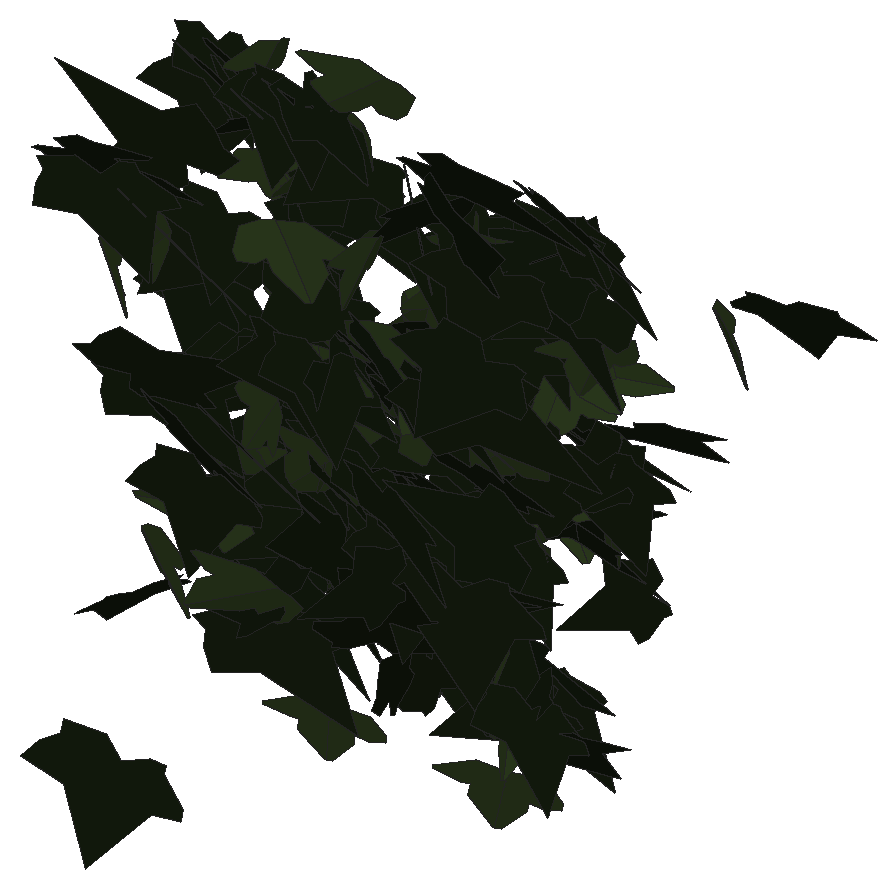
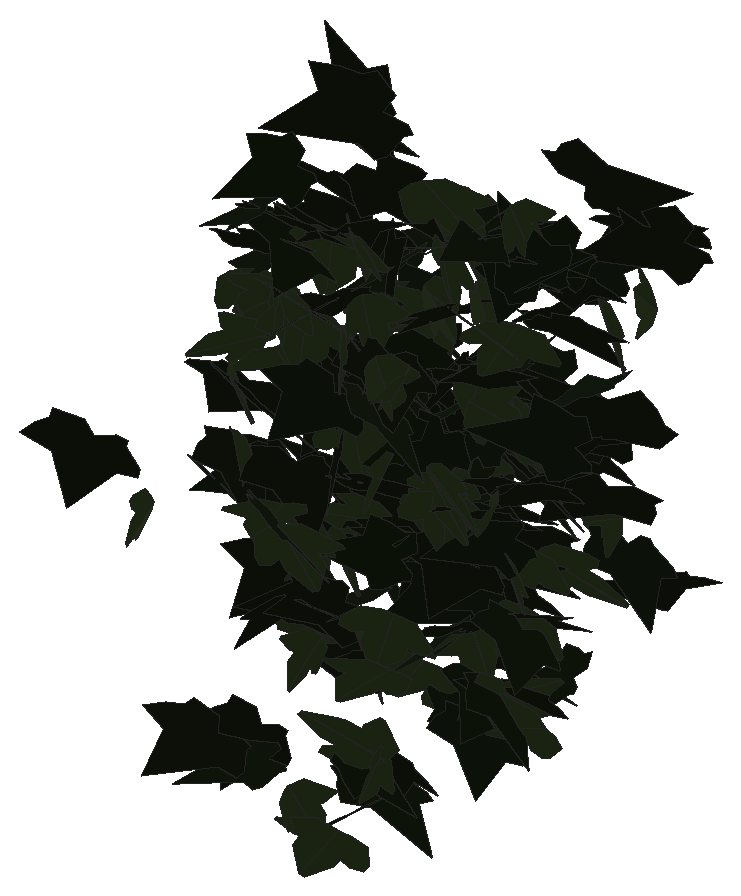
# SketchUp Ruby script. Lengths in millimetres.
U = 1.mm
M = Sketchup.active_model
def pt(a) = Geom::Point3d.new(a.map { |v| v * U })
def face(e, loops, mat)
  f = e.add_face(loops[0].map { |a| pt(a) })
  loops[1..].each { |l| e.add_face(l.map { |a| pt(a) }).erase! }
  f.material = f.back_material = mat if mat
  f
end
# faces: each face lists its corners as indices into pts; further lists are holes
def faces(e, pts, list, mat = nil) = list.each { |f| face(e, (f[0].is_a?(Array) ? f : [f]).map { |l| l.map { |i| pts[i] } }, mat) }
# xy, xz, yz: faces in a plane at the given z, y or x. An outline is a flat list of corners, or four numbers for a rectangle; further outlines are holes
def ring(l) = l.size == 4 ? [[l[0], l[1]], [l[2], l[1]], [l[2], l[3]], [l[0], l[3]]] : l.each_slice(2).to_a
def flat(e, list, mat, &to3) = list.each { |f| face(e, (f[0].is_a?(Array) ? f : [f]).map { |l| ring(l).map { |u, v| to3.(u, v) } }, mat) }
def xy(e, z, list, mat = nil) = flat(e, list, mat) { |x, y| [x, y, z] }
def xz(e, y, list, mat = nil) = flat(e, list, mat) { |x, z| [x, y, z] }
def yz(e, x, list, mat = nil) = flat(e, list, mat) { |y, z| [x, y, z] }
def lines(e, pts, list) = list.each { |a, b| e.add_line(pt(pts[a]), pt(pts[b])) }
# prism: a flat outline (further loops are holes) pulled along v
def prism(e, loops, v, mat = nil)
  f = face(e, loops, mat); d = Geom::Vector3d.new(v.map { |x| x * U })
  f.pushpull(f.normal.samedirection?(d) ? d.length : -d.length)
end
def box(e, o, s, mat = nil) = prism(e, [[o, [o[0] + s[0], o[1], o[2]], [o[0] + s[0], o[1] + s[1], o[2]], [o[0], o[1] + s[1], o[2]]]], [0, 0, s[2]], mat)
def at(x, y, z, deg = 0) = Geom::Transformation.translation(pt([x, y, z])) * Geom::Transformation.rotation(ORIGIN, Z_AXIS, deg.degrees)
def axes(o, x, y, z) = Geom::Transformation.new([*x, 0, *y, 0, *z, 0, *pt(o).to_a, 1])
def part(name) = M.definitions.add(name)
# library, detail: a bought-in or finely detailed component or shape, given as its bounding box
def library(name, o, s) = part(name).tap { |d| box(d.entities, o, s) }
def detail(e, o, s) = box(e.add_group.entities, o, s)
def put(e, d, t, mat = nil) = e.add_instance(d, t).tap { |i| i.material = mat if mat }
def group(e, t, mat = nil) = e.add_group.tap { |g| g.transformation = t; g.material = mat if mat }.entities
root = M.entities
M.materials.add("efeu1").color = [18, 25, 13]
M.materials.add("efeu2").color = [43, 57, 29]
c1 = part("ivyleaf_10")
p = [[0,12.8,-0.8],[-1.5,51.3,-10.9],[-4.9,51,-11.6],[-13.6,26.5,-7.3],[-13.2,15.9,-4.6],[-21.1,19.3,-7.2],
  [-29.5,16.3,-8.3],[-29.2,8.3,-6.2],[-19.7,-9.8,0.5],[-7.6,-13,4],[1,-12.2,5.8],[-0.4,51.1,-11.1],
  [-1.5,51.1,-10.9],[1,-12.4,5.9],[16.9,-12.4,3.5],[35.1,9.1,-5.1],[35,12.9,-6.1],[20.5,16.4,-4.9],
  [15.8,15,-3.8],[15.3,27.6,-7.1],[12.8,31.3,-7.8]]
faces(c1.entities,p,[[0,1,2,3,4,5,6,7,8,9,10],[11,12,0,13,14,15,16,17,18,19,20]],"efeu2")
c2 = part("ivyleaf_9")
p = [[39.1,54.8,31.7],[34.5,51.8,30.2],[-5.3,25.2,17.3],[-17.9,28.3,20.9],[-21.6,21.7,17],[-20.2,4.3,5.3],
  [-22.9,-0.3,2.5],[-17.1,-4,-0.6],[-2,-2.1,-1.2],[-0.7,-15.4,-10.1],[16.6,-22.3,-16.7],[21.1,-15.1,-12.5],
  [32.7,-10.7,-11],[46.1,-1.8,-6.6],[30.8,11.2,3.8]]
faces(c2.entities,p,[[0,1,2,3,4,5,6,7,8,9,10,11,12,13,14]],"efeu1")
put(root,c1,axes([6232.5,1056.6,3614.3],[-0.05301,-0.61059,-0.9805],[0.31818,0.96833,-0.60776],[2.1752,-0.15652,0.06501]))
put(root,c2,axes([6249.3,764.1,3661.4],[0.62349,1.03972,0.40292],[-0.08884,0.43237,-1.07776],[-2.12033,0.28762,0.16364]))
put(root,c2,axes([6209.3,719.3,3591.9],[1.27144,-0.98934,0.14029],[0.12142,-0.12619,-1.19365],[1.89788,0.67086,-0.01762]))
put(root,c2,axes([6208.7,511.3,4104.5],[2.12507,0.22385,0.53376],[0.99329,0.11205,-1.13878],[-0.47626,1.23251,0.00658]))
put(root,c2,axes([6232.9,713.1,4143.1],[0.08178,-1.24795,-0.07814],[-0.03089,0.07763,-1.24862],[2.37956,0.04389,-0.01352]))
put(root,c2,axes([6218.2,708.4,3903.7],[1.22381,0.07724,1.11184],[1.74203,0.69576,-0.57771],[-1.21021,1.07962,0.29276]))
put(root,c2,axes([6249.1,685.7,3888.7],[-1.16287,-1.04199,0.06481],[0.13254,-0.11561,-1.20211],[1.98252,-0.60346,0.11838]))
put(root,c1,axes([6275.1,773.1,3563.5],[0.97003,0.62714,0.84354],[-1.0128,-0.6545,0.80813],[1.72518,-0.73686,0.00013]))
put(root,c2,axes([6228.3,627.8,3807.5],[-0.63659,-0.70921,-1.06674],[1.06415,0.9111,-0.78106],[2.19345,-0.64785,0.06934]))
put(root,c1,axes([6217.4,778.9,3544.9],[1.27917,-0.07652,0.94431],[1.79881,0.13391,-0.66186],[-0.1242,1.15131,0.13975]))
put(root,c2,axes([6258.2,1022.9,3608.5],[-1.9163,-0.03935,-0.6563],[1.24656,0.04446,-1.00753],[0.10893,-1.20107,-0.0158]))
put(root,c1,axes([6272.5,569.3,4006.5],[0.92456,-0.93891,-0.66939],[-0.43427,0.63373,-1.05449],[2.15118,0.53147,0.07482]))
put(root,c2,axes([6261.3,690.1,4122.7],[-1.8784,-0.64082,-0.43417],[0.80372,0.14384,-1.17228],[1.23462,-1.06861,0.10257]))
put(root,c2,axes([6282,772.7,3572.1],[-0.28697,1.1485,-0.09498],[0.04934,-0.09239,-1.15827],[-2.19272,-0.15238,-0.01363]))
put(root,c2,axes([6286.9,742.7,3658.5],[-1.79291,-0.44896,0.52127],[-0.65172,-0.46059,-1.01555],[1.13559,-0.97316,0.24017]))
put(root,c2,axes([6283.4,1045,3602.5],[-0.96373,0.75103,-0.72225],[0.4298,-0.70483,-0.89125],[-1.93594,-0.53035,0.16168]))
put(root,c1,axes([6302.6,629.6,3679],[0.87197,-0.10124,-1.08289],[-1.99972,0.26228,-0.46907],[0.5346,1.1462,0.01169]))
put(root,c1,axes([6260.9,740.5,3660.5],[-2.08189,0.17325,-0.34606],[0.63339,-0.10845,-1.10628],[-0.37593,-1.14219,0.05255]))
put(root,c1,axes([6272.1,757.5,3744.2],[1.12472,-1.03315,-0.04774],[0.08934,0.08172,-1.18745],[1.96635,0.58723,0.08126]))
put(root,c2,axes([6274.2,720.4,3839.9],[-1.10481,-1.02823,0.31517],[-0.2383,-0.2911,-1.18032],[2.03287,-0.59294,0.03293]))
put(root,c1,axes([6253.6,514.3,4002.3],[-0.29737,0.54425,-1.13301],[0.71097,-1.07003,-0.56551],[-2.28413,-0.40392,-0.02852]))
put(root,c2,axes([6250.1,666.7,4146],[2.24581,-0.45086,-0.2997],[-0.51361,0.1332,-1.26292],[0.89322,1.21017,0.02735]))
put(root,c2,axes([6262.3,633.6,3925.4],[-0.58984,-1.05015,0.63585],[0.11524,-0.66807,-1.07386],[2.33362,-0.23244,0.21375]))
put(root,c2,axes([6270.5,771.7,3577.5],[-1.45641,-0.65826,-0.57461],[0.85524,0.35858,-1.00924],[1.42619,-0.88724,0.01843]))
put(root,c1,axes([6253.9,1055.6,3623.5],[-0.9404,-0.48923,0.92476],[1.29808,0.62487,0.69501],[-1.50983,0.84195,0.02154]))
put(root,c1,axes([6260.3,1115.5,3524.7],[2.02857,0.20437,0.47791],[0.70398,0.46776,-1.025],[-0.69497,1.07036,0.35669]))
put(root,c2,axes([6262.4,491.6,4101.6],[-0.88382,-0.92601,-0.72646],[0.85052,0.58375,-1.02977],[2.07225,-0.63454,0.11281]))
put(root,c2,axes([6299.4,495.2,3642.6],[0.21417,1.25654,-0.14344],[-0.03367,-0.14242,-1.26156],[-2.40674,0.11381,0.00488]))
put(root,c2,axes([6246.5,565.1,3841.8],[0.08093,-0.25758,1.32814],[2.51797,-0.26974,-0.09467],[0.53802,1.30115,0.24329]))
put(root,c2,axes([6278.9,727.1,3837.3],[-1.05285,-0.9828,-0.49121],[0.82274,0.31091,-1.1089],[1.92242,-0.67131,0.20556]))
put(root,c2,axes([6341.6,517.9,4138.5],[-0.04794,0.02741,1.38699],[-2.13929,0.8126,-0.03647],[-1.54735,-1.12431,0.00745]))
put(root,c2,axes([6304,773.3,3510.7],[0.68411,1.10542,0.12641],[-0.015,0.13537,-1.16136],[-2.1175,0.35618,0.04906]))
put(root,c2,axes([6318.5,613.4,4000.6],[-2.21471,-0.36537,0.03234],[-0.0571,-0.0124,-1.21968],[0.69574,-1.16406,0.00284]))
put(root,c2,axes([6300.2,745.1,3705.3],[-1.90049,-0.35101,-0.50364],[0.92645,0.13317,-1.05797],[0.71185,-1.11043,0.03232]))
put(root,c2,axes([6285.9,1050.6,3522.3],[-0.00059,-1.1861,0.07634],[-0.02876,-0.07633,-1.18601],[2.26188,-0.00128,-0.01506]))
put(root,c2,axes([6325.9,673.5,3826.8],[-2.07058,0.44277,-0.26856],[0.47756,-0.09588,-1.17458],[-0.86215,-1.11649,-0.00563]))
put(root,c2,axes([6345.5,732.4,3594.6],[-1.88833,0.31067,0.52272],[-0.92657,0.1935,-1.0391],[-0.69339,-1.10464,-0.03501]))
put(root,c2,axes([6269.8,708.5,4118.2],[2.25595,-0.48028,-0.56029],[1.04081,-0.14012,1.27708],[-0.94304,-1.30358,0.06916]))
put(root,c1,axes([6300.3,719.8,4032.5],[-1.77868,-0.71839,-0.39001],[0.91882,-0.00703,-1.1439],[1.25543,-1.01266,0.28462]))
put(root,c2,axes([6310.8,744.9,3549.7],[0.75041,0.9439,0.60512],[0.35622,0.57703,-1.02204],[-2.10394,0.43436,0.04278]))
put(root,c1,axes([6306.3,693,3710.8],[-2.12167,-0.29345,-0.3124],[0.59799,0.03256,-1.15182],[0.55482,-1.15728,0.04681]))
put(root,c1,axes([6312,775.4,3632.8],[1.17688,0.9457,-0.28185],[-0.5072,-0.16021,-1.12226],[-1.8083,0.66042,0.13134]))
put(root,c1,axes([6314.7,689.2,4175.6],[-0.25923,-1.20094,0.332],[0.19943,-0.34384,-1.20076],[2.36296,-0.10273,0.13776]))
put(root,c2,axes([6276.5,752,3774.6],[2.17748,-0.26341,0.18836],[0.33859,-0.06662,-1.17379],[0.51497,1.1576,-0.02469]))
put(root,c2,axes([6342.1,928.3,3495.4],[-0.01489,1.13626,-0.24426],[-0.89474,-0.22648,-1.03851],[-2.02289,0.09181,0.46114]))
put(root,c1,axes([6307.4,751.8,3806.7],[-0.32943,1.14607,-0.2796],[0.04214,-0.27939,-1.15891],[-2.24478,-0.17343,0.01927]))
put(root,c1,axes([6325.1,1101.8,3551.6],[-0.34351,-1.11285,0.38624],[-0.00678,-0.39023,-1.12601],[2.2419,-0.1717,0.05578]))
put(root,c2,axes([6281.2,536.1,4046.4],[1.4568,-0.93345,0.51682],[0.63787,-0.39351,-1.20713],[1.92789,0.83556,0.00886]))
put(root,c2,axes([6319,617.5,4021.5],[-0.72037,-1.14315,0.21033],[-0.13577,-0.19794,-1.20417],[2.20799,-0.38513,-0.00542]))
put(root,c2,axes([6330.6,667,4115.8],[1.101,1.10722,0.09654],[0.07566,0.08815,-1.24923],[-2.11391,0.57984,0.00557]))
put(root,c1,axes([6309.9,517.9,3690.6],[-0.95877,0.74151,-0.88779],[0.83749,-0.77267,-0.89506],[-2.03595,-0.66703,0.0499]))
put(root,c2,axes([6338.6,752.5,3787.1],[-1.60733,-0.82833,-0.18309],[0.36491,0.06528,-1.17978],[1.57275,-0.86169,0.08662]))
put(root,c2,axes([6362.7,672.8,3674.6],[-1.9795,-0.59,0.39192],[-0.65357,-0.18893,-1.19577],[1.17902,-1.09531,-0.00485]))
put(root,c2,axes([6345,774.3,3638.7],[-0.9698,-1.0459,0.04124],[0.04507,-0.05737,-1.1625],[1.99159,-0.508,0.04639]))
put(root,c2,axes([6309.1,545.4,3811.1],[1.01793,-0.74557,0.84956],[0.85177,-0.72337,-0.91658],[1.9754,0.6961,-0.04256]))
put(root,c1,axes([6359.5,700.7,4056.8],[-0.0824,-1.22848,-0.26768],[-0.06577,0.2689,-1.22849],[2.39199,-0.03493,-0.043]))
put(root,c2,axes([6344.7,675.1,4139.3],[-0.71835,-1.16583,0.13824],[-0.10992,-0.1266,-1.2253],[2.23165,-0.38151,-0.01585]))
put(root,c1,axes([6359.6,700.8,3901.9],[-0.42811,-0.75898,0.99529],[0.03203,-1.01298,-0.76866],[2.38195,-0.12279,0.18922]))
put(root,c1,axes([6380,757.4,3822.3],[0.79364,-0.5299,-0.96676],[-1.16785,0.74714,-0.67421],[1.74315,0.74182,-0.01154]))
put(root,c2,axes([6326.9,730.9,3684.3],[1.85925,-0.6502,-0.05486],[-0.10712,0.01444,-1.17335],[1.23722,0.97834,-0.01915]))
put(root,c1,axes([6349.7,719,3696.6],[-2.10011,-0.11334,-0.39142],[0.77218,-0.20025,-1.08581],[0.07229,-1.15358,0.22694]))
put(root,c2,axes([6354.3,747.7,3723],[1.97838,0.39973,-0.36048],[-0.64775,-0.11925,-1.11366],[-0.79365,1.09375,0.01033]))
put(root,c1,axes([6394.9,754.1,3806.4],[-1.49231,0.27745,0.8565],[-1.5876,0.20341,-0.82956],[-0.64463,-1.14326,0.06026]))
put(root,c2,axes([6395.1,688.1,4006.1],[0.2398,0.73833,0.99377],[-1.25297,0.88592,-0.57473],[-1.99545,-0.46755,0.48031]))
put(root,c2,axes([6343.1,776,3631],[1.3619,-0.63693,-0.66418],[-0.53594,0.64944,-0.92618],[1.66737,0.72899,0.2448]))
put(root,c2,axes([6352.5,668.6,4137.1],[1.40171,0.63723,0.79432],[0.57405,0.79981,-0.92129],[-1.85114,0.73054,0.31578]))
put(root,c2,axes([6343,713.3,3987.7],[0.61839,-1.16376,-0.32096],[-0.07963,0.32133,-1.20745],[2.29618,0.32456,0.04457]))
put(root,c2,axes([6338.8,769.9,3532.9],[0.51879,-0.89059,0.71161],[0.42236,-0.67621,-0.93131],[2.12809,0.35132,0.01136]))
put(root,c1,axes([6379.5,754.8,3785.1],[-1.97198,-0.54972,0.0504],[-0.08195,-0.02636,-1.17293],[1.04741,-1.03703,0.0031]))
put(root,c2,axes([6368.7,383.8,3521.1],[-1.4246,-1.25737,0.03019],[-0.02962,-0.02587,-1.46331],[2.39353,-0.74869,-0.00014]))
put(root,c2,axes([6366.9,524.2,3780.6],[-1.96974,-0.27354,-0.73194],[1.38995,0.09326,-1.06754],[0.52874,-1.26419,0.07962]))
put(root,c2,axes([6361.5,679.2,4142],[-0.33676,-1.16768,0.36339],[0.22932,-0.38204,-1.16892],[2.31614,-0.13195,0.16857]))
put(root,c2,axes([6375.1,689.4,3832.4],[-0.91054,-0.05091,1.13101],[0.10556,-1.22742,-0.03179],[2.15212,0.03867,0.48008]))
put(root,c2,axes([6402.9,683.2,3931.5],[-1.91895,-0.64966,0.29713],[-0.40501,-0.21748,-1.19766],[1.29788,-1.0284,0.06557]))
put(root,c1,axes([6425,729.5,3765.6],[0.67534,0.16747,-1.12453],[-2.06941,0.39415,-0.28441],[0.63215,1.11137,0.27032]))
put(root,c1,axes([6391.5,589.5,3842.8],[1.44432,-0.96288,-0.33665],[-0.22499,0.33376,-1.22107],[1.92825,0.76017,0.10969]))
put(root,c1,axes([6394.6,707.9,3790.8],[0.03269,-1.10472,-0.47812],[0.18426,0.47789,-1.1007],[2.28354,-0.02275,0.09566]))
put(root,c1,axes([6399.1,705.8,3674.1],[0.08549,-1.17309,0.03024],[-0.02074,-0.03068,-1.17388],[2.23326,0.04462,-0.01206]))
put(root,c2,axes([6369.5,681.2,4150.1],[0.89883,-1.11192,-0.44039],[-0.17361,0.43862,-1.20526],[2.26951,0.47392,0.08222]))
put(root,c2,axes([6371.2,684.3,3763.8],[0.31078,-1.15416,0.38697],[0.20438,-0.37526,-1.16454],[2.30774,0.18866,0.05102]))
put(root,c1,axes([6431.3,704.7,4174.5],[-1.73617,-0.42045,0.7532],[-1.19273,-0.43024,-0.9992],[1.1281,-1.10199,0.10274]))
put(root,c1,axes([6421.4,1003,3832.9],[-1.47331,-0.79521,0.40229],[-0.55209,-0.27901,-1.10971],[1.60371,-0.82659,-0.01244]))
put(root,c2,axes([6375.4,718.4,3650.3],[2.04658,0.33696,0.32128],[0.53682,0.17182,-1.12429],[-0.70496,1.10907,0.07657]))
put(root,c2,axes([6381.9,697.6,3674.5],[-0.71118,-0.70522,-0.99888],[0.80653,0.90505,-0.79751],[2.18288,-0.56416,-0.03077]))
put(root,c2,axes([6372.6,1106,3590.8],[2.02981,-0.48671,-0.23478],[-0.01487,0.50552,-1.08345],[1.02834,0.96801,0.44776]))
put(root,c1,axes([6415.4,662.2,3471.5],[-2.08781,-0.40835,0.09557],[-0.1608,-0.04696,-1.17044],[0.7818,-1.10015,0.01448]))
put(root,c1,axes([6404.3,713.4,4103.5],[1.63278,-0.86703,-0.27942],[0.03187,0.39878,-1.18597],[1.73342,0.80936,0.285]))
put(root,c2,axes([6441.8,674.4,3746.6],[-2.05619,-0.45228,0.729],[-1.27776,-0.28408,-1.17123],[1.01648,-1.272,0.00237]))
put(root,c1,axes([6437,625.3,3778.1],[-1.80419,0.22178,0.68669],[-1.31132,0.05878,-0.97016],[-0.4082,-1.16908,0.08149]))
put(root,c2,axes([6412.9,615.5,3879],[0.82511,-1.18761,-0.69133],[0.4202,-0.6553,1.26418],[-2.58136,-0.48628,-0.01519]))
put(root,c2,axes([6384.9,713.9,4042],[0.29901,-1.07885,-0.60291],[0.28765,0.61997,-1.07],[2.33449,0.06179,0.20907]))
put(root,c2,axes([6412.2,713.4,3852.7],[1.7619,-0.09633,-0.76545],[-1.4253,0.17504,-0.92776],[0.35275,1.18841,0.0746]))
put(root,c2,axes([6411.4,1070,3607.6],[2.06853,0.01255,-0.51831],[-0.98673,0.01986,-1.08669],[-0.00529,1.20397,0.02333]))
put(root,c2,axes([6434.4,691.7,4096.6],[-1.73442,-0.67348,0.51749],[-0.27302,-0.62605,-1.0674],[1.59323,-0.84045,0.38043]))
put(root,c2,axes([6386,519.7,3853.7],[1.86849,-0.79741,0.12429],[0.19887,-0.06849,-1.26473],[1.52302,0.98723,0.01266]))
put(root,c1,axes([6425.8,801.5,3625],[-2.19935,-0.0944,-0.0961],[0.18266,0.00549,-1.15945],[0.17991,-1.15958,0.00233]))
put(root,c2,axes([6398.2,637.9,3613.2],[0.93623,-1.17285,-0.11904],[-0.06194,0.11542,-1.27175],[2.24277,0.49279,0.01457]))
put(root,c1,axes([6429.8,645,3787.6],[0.36199,-0.93641,-0.81977],[0.19376,0.83821,-0.93386],[2.36066,0.07479,0.20235]))
put(root,c1,axes([6433.2,686.2,3651.2],[-0.05527,-1.13651,-0.47139],[0.1245,0.46942,-1.13581],[2.33836,-0.05186,0.04933]))
put(root,c1,axes([6407.2,765,3558],[2.00634,0.29448,0.43772],[0.7854,0.14904,-1.09413],[-0.62551,1.13168,0.0302]))
put(root,c2,axes([6382.1,695.5,3680.8],[1.48132,-0.17336,0.99952],[1.84203,-0.25047,-0.79712],[0.57834,1.24181,-0.02124]))
put(root,c2,axes([6461.8,1002.5,3863.5],[-1.68716,0.77661,-0.13606],[0.18098,-0.09793,-1.1785],[-1.4896,-0.8915,0.01093]))
put(root,c2,axes([6482.2,696.3,3656],[-0.67156,0.28688,1.16377],[-1.83672,0.65147,-0.45321],[-1.35289,-1.02687,0.0376]))
put(root,c1,axes([6417.7,636.1,3883],[2.19798,-0.21825,0.33949],[0.65918,0.00766,-1.1733],[0.39433,1.20373,0.06902]))
put(root,c1,axes([6417.6,581.8,4048.3],[1.94868,0.57797,0.36175],[0.48874,0.27772,-1.17056],[-1.20214,1.04981,0.1105]))
put(root,c1,axes([6412.6,835.3,3575.9],[1.37454,0.69786,0.59073],[0.84148,0.39235,-1.00406],[-1.52313,0.84654,-0.02161]))
put(root,c1,axes([6477.9,471.8,3718.6],[-1.5218,-0.36728,0.91799],[-1.61395,-0.35231,-0.87961],[0.96758,-1.16531,-0.0234]))
put(root,c1,axes([6452.4,679.5,4014.1],[0.23806,-1.17731,0.40735],[0.1893,-0.39866,-1.18272],[2.36343,0.15052,0.0537]))
put(root,c2,axes([6439.5,647.9,3749.1],[1.49479,-0.95257,-0.33443],[0.43637,-0.24434,1.23443],[-1.8712,-0.81793,0.02072]))
put(root,c2,axes([6488.3,488,3704],[-1.24645,1.12217,0.18453],[-0.21677,0.14715,-1.29909],[-2.15352,-0.66432,0.02396]))
put(root,c2,axes([6447.8,609,3903.2],[-0.40144,-1.28899,-0.02219],[0.00169,0.02234,-1.30613],[2.45358,-0.21091,-0.00273]))
put(root,c2,axes([6443.2,1114.6,3605.8],[1.93199,0.56622,0.29144],[0.35269,0.26204,-1.15457],[-1.15954,1.02311,0.13441]))
put(root,c2,axes([6454.3,616.5,3899],[0.80917,-0.73412,-1.04501],[-0.98973,0.90644,-0.84835],[2.21995,0.67171,0.00268]))
put(root,c2,axes([6436.6,530.6,3637.7],[-0.44383,-0.83855,-1.07303],[1.14699,0.9127,-0.84423],[2.32421,-0.61054,0.21171]))
put(root,c2,axes([6496.8,738,3878.1],[-0.49954,1.15079,0.26935],[-0.43296,0.22156,-1.16829],[-2.20731,-0.3039,0.1682]))
put(root,c1,axes([6473.4,751.4,3808.2],[-0.48642,0.90949,0.72909],[-0.49831,0.68254,-0.94321],[-2.16177,-0.36198,0.05336]))
put(root,c1,axes([6465.9,731.6,3918.1],[-0.19377,1.22145,0.02751],[-0.0016,0.02753,-1.22568],[-2.32525,-0.1018,-0.00145]))
put(root,c1,axes([6485.5,738.3,3926.3],[-0.33376,-1.20364,0.01617],[-0.02016,-0.0148,-1.21632],[2.29088,-0.17549,-0.00835]))
put(root,c2,axes([6512.3,751.9,3772.8],[-2.0331,-0.18471,0.47145],[-0.80005,-0.29007,-1.06616],[0.5372,-1.13105,0.19644]))
put(root,c2,axes([6438.6,769.2,3697.9],[1.66133,-0.6159,0.48853],[0.83933,-0.22067,-1.06621],[1.23855,0.97568,0.06724]))
put(root,c2,axes([6530,536.7,3755.9],[0.35588,-0.00986,-1.45147],[-2.76141,0.03981,-0.18719],[0.07754,1.46292,-0.00468]))
put(root,c2,axes([6499.6,707.5,3925.7],[0.72628,1.15016,-0.07246],[-0.06728,-0.06461,-1.21174],[-2.19229,0.38302,0.01318]))
put(root,c2,axes([6477.3,758.1,3549.9],[-0.53131,-1.11605,-0.265],[0.26461,0.2378,-1.14798],[2.16703,-0.30267,0.07521]))
put(root,c1,axes([6496,859.7,3596],[0.34903,0.74373,0.8887],[-0.44585,0.90498,-0.70901],[-2.15999,-0.06662,0.28995]))
put(root,c1,axes([6511.8,738.6,3535.7],[0.75796,-1.13674,-0.19511],[-0.12377,0.18395,-1.20449],[2.1916,0.40353,-0.00054]))
put(root,c2,axes([6480.8,677.8,3737.4],[2.2573,-0.10363,-0.0657],[-0.12367,0.01105,-1.19056],[0.19808,1.18782,0.00534]))
put(root,c2,axes([6466.6,728.9,3832.5],[1.16356,-0.79804,0.71074],[0.95148,-0.51012,-1.00281],[1.79758,0.78658,0.07074]))
put(root,c2,axes([6475,643.6,3768.3],[1.6226,-0.87466,0.2312],[0.2958,-0.17136,-1.22141],[1.69624,0.86658,-0.00817]))
put(root,c2,axes([6473.8,635,3913.1],[1.71916,-0.72708,0.40505],[0.58616,-0.26333,-1.15951],[1.47158,0.9543,-0.01134]))
put(root,c1,axes([6527.9,741.7,3832.3],[-1.73834,-0.76601,0.12842],[-0.16849,-0.09427,-1.19197],[1.46857,-0.91753,0.01525]))
put(root,c2,axes([6471,714.5,3692.8],[0.54453,-0.38955,1.27046],[1.68241,-0.91452,-0.47949],[1.88828,0.92714,0.06084]))
put(root,c2,axes([6535.2,760.4,3816.6],[0.57573,-0.0139,-1.14852],[-1.79141,0.67767,-0.25612],[1.25282,0.97538,0.16157]))
put(root,c2,axes([6535.9,663.3,4016.8],[0.08852,-0.67229,1.10508],[0.27732,1.10148,0.66397],[-2.44614,0.10054,0.11527]))
put(root,c1,axes([6505,620.3,3947.3],[-1.71916,0.4476,-0.76053],[1.09962,-0.52265,-0.99384],[-1.26948,-1.05886,0.16906]))
put(root,c2,axes([6507.4,614.1,3794.7],[0.08557,-1.1658,0.27314],[0.06474,-0.27198,-1.16644],[2.27791,0.05152,0.02289]))
put(root,c1,axes([6528.6,577,4075.3],[-0.00593,-1.19004,0.44421],[0.26777,-0.4418,-1.1826],[2.40265,0.0463,0.13289]))
put(root,c1,axes([6536.1,703.4,3979.3],[-0.5936,-1.20336,0.01364],[0.18075,-0.03865,-1.23896],[2.28324,-0.30979,0.10163]))
put(root,c2,axes([6492,748.9,3515],[1.24455,-0.73237,0.65307],[0.81693,-0.49224,-0.98181],[1.67938,0.78219,-0.00638]))
put(root,c2,axes([6515.4,685.3,4035.9],[0.09533,-1.23206,0.26626],[-0.0573,-0.26756,-1.23243],[2.3983,0.04258,-0.04003]))
put(root,c1,axes([6526.8,704.7,3914.8],[1.6273,-0.82679,0.25427],[0.58183,-0.04562,-1.17634],[1.54004,0.89087,0.17574]))
put(root,c1,axes([6545.2,736.6,3948.5],[0.6312,-1.04789,-0.51734],[0.22572,0.56517,-1.06875],[2.21267,0.24127,0.2566]))
put(root,c2,axes([6583.8,658.3,3894.7],[-1.1175,0.96709,0.40811],[-0.71734,0.24218,-1.11618],[-1.86451,-0.6728,0.18483]))
put(root,c2,axes([6544.2,595.8,3567.7],[-0.0179,-0.5434,1.30663],[1.22245,1.16266,0.48815],[-2.39984,0.5963,0.23892]))
put(root,c2,axes([6583.1,624.3,3580.8],[-0.34783,0.95519,1.06688],[-0.29998,1.05558,-0.97208],[-2.70882,-0.23955,-0.02934]))
put(root,c1,axes([6518.4,706.8,3694.1],[-0.8829,0.13468,-1.0838],[1.99776,-0.27011,-0.48287],[-0.57386,-1.14755,-0.01354]))
put(root,c2,axes([6577.6,629.2,4120.4],[-0.46706,0.85466,-0.86252],[0.06274,-0.87494,-0.87636],[-2.3101,-0.19656,0.15058]))
put(root,c2,axes([6532.7,600.6,3942.2],[0.16455,-0.94849,0.9769],[0.30837,-0.96475,-0.95103],[2.57299,0.17628,0.0515]))
put(root,c2,axes([6541.9,741.6,3855.7],[0.0664,-0.46323,1.1072],[0.37183,-1.0907,-0.46249],[2.25376,0.19359,0.04368]))
put(root,c2,axes([6552.3,753.8,3880.1],[1.71817,0.72377,0.29673],[0.37405,0.22871,-1.15584],[-1.44099,0.92236,0.05377]))
put(root,c1,axes([6558.5,695.2,4063.7],[1.45045,-0.91244,0.40984],[0.56056,-0.2877,-1.1882],[1.81929,0.8161,0.03936]))
put(root,c2,axes([6562.6,615.5,3736.7],[1.48065,-1.04611,-0.25855],[0.31019,-0.20099,1.30364],[-2.02727,-0.7948,0.01063]))
put(root,c2,axes([6546.3,709.7,3571.1],[0.26842,-1.19412,0.29819],[0.22896,-0.28533,-1.19952],[2.33122,0.16552,0.08347]))
put(root,c2,axes([6603,616.9,3753],[-2.33443,-0.3044,0.27362],[-0.48755,-0.10322,-1.26323],[0.60754,-1.25248,0.03761]))
put(root,c1,axes([6611.7,700.3,3825.4],[-1.94209,0.15526,0.7213],[-1.36036,0.09726,-1.03213],[-0.34824,-1.24583,0.00931]))
put(root,c2,axes([6581.7,700.7,4072.5],[-1.20578,-1.14175,0.20824],[-0.17858,-0.18608,-1.30572],[2.20159,-0.64041,0.00813]))
put(root,c1,axes([6598.7,696.8,4048.7],[-2.27915,-0.39134,-0.00449],[0.01441,-0.00871,-1.25981],[0.7447,-1.19751,0.01063]))
put(root,c1,axes([6588.4,755.7,3687.6],[1.72933,-0.75502,-0.17753],[0.13739,0.35458,-1.13854],[1.46973,0.85523,0.31532]))
put(root,c2,axes([6630.2,723.9,3858.4],[-1.86117,0.66456,0.19935],[-0.26644,0.14843,-1.18155],[-1.2933,-0.98693,-0.04346]))
put(root,c2,axes([6607,752.8,3761.1],[0.8239,1.00584,-0.46759],[-0.34711,-0.43056,-1.09504],[-2.08233,0.46975,-0.00247]))
put(root,c1,axes([6614,672.2,3627.3],[1.13116,-0.83326,-0.75214],[-0.69836,0.66008,-1.02124],[2.019,0.69516,0.06815]))
put(root,c2,axes([6563.8,720.2,3572.6],[0.10173,0.10975,-1.2024],[1.41716,0.94445,0.1193],[1.8089,-0.74609,-0.02585]))
put(root,c1,axes([6608.9,733.8,3949.4],[-2.16041,-0.3909,-0.04214],[0.07183,0.01983,-1.20055],[0.74481,-1.13576,-0.00646]))
put(root,c2,axes([6572.8,664.6,3652.1],[-0.26723,-1.03973,-1.01108],[0.91987,0.92419,-1.0175],[2.60239,-0.43344,0.25583]))
put(root,c2,axes([6559.5,633.8,3669.5],[0.27079,-0.13325,1.28343],[2.31776,-0.41287,-0.17787],[0.81162,1.22351,0.07975]))
put(root,c2,axes([6639.8,717.5,3534.6],[-2.18046,-0.08665,0.29386],[-0.56015,-0.00458,-1.14883],[0.16192,-1.18276,-0.01708]))
put(root,c2,axes([6643.9,741.2,3983],[-2.20594,0.35504,0.07558],[-0.2672,-0.20526,-1.18885],[-0.63709,-1.14325,0.23692]))
put(root,c2,axes([6600,658.3,3815.3],[2.15852,0.1277,-0.38192],[-0.742,0.06236,-1.13692],[-0.19192,1.1951,0.10014]))
put(root,c2,axes([6602.6,555.9,3757.1],[-0.49127,-1.36165,0.55677],[-0.13922,-0.5527,-1.3856],[2.79631,-0.26674,0.02883]))
put(root,c1,axes([6601.4,797.6,3721.7],[1.29092,0.94599,0.19596],[0.2842,0.1339,-1.16325],[-1.81654,0.69322,-0.04273]))
put(root,c2,axes([6569.9,541.5,3716.1],[1.1819,-0.04175,1.2435],[2.34371,0.21904,-0.60764],[-0.33807,1.37258,0.13479]))
put(root,c1,axes([6603.3,558.7,3906.2],[0.09923,-0.0986,-1.2203],[1.12748,1.07092,-0.06122],[2.03909,-0.58735,0.09323]))
put(root,c1,axes([6616.2,1034.3,3820.6],[-0.91911,1.08305,-0.0953],[0.07215,-0.08744,-1.18584],[-2.06797,-0.48441,0.00098]))
put(root,c2,axes([6603.9,740.2,3963.6],[0.28098,-1.20141,-0.09832],[-0.0462,0.09607,-1.21038],[2.2937,0.14911,-0.01234]))
put(root,c2,axes([6607.7,714.5,3701.4],[0.08264,-1.18127,-0.1517],[-0.03906,0.15104,-1.18197],[2.26632,0.04568,-0.01484]))
put(root,c2,axes([6598.3,582.5,3952.1],[1.40939,-1.03022,-0.2197],[-0.23804,0.18067,-1.26875],[1.99062,0.75101,0.00384]))
put(root,c2,axes([6611.4,492.2,3700.1],[2.10071,0.62926,0.69494],[-1.21546,-0.2812,1.26898],[1.30623,-1.27366,0.06318]))
put(root,c2,axes([6614.9,683.4,3961.4],[-0.68447,-1.19282,-0.28092],[0.11247,0.27555,-1.24566],[2.32958,-0.36378,-0.0224]))
put(root,c2,axes([6635.9,698.7,4041.6],[0.92326,1.03783,0.50874],[0.28284,0.49114,-1.14365],[-2.18148,0.50292,0.06703]))
put(root,c1,axes([6652.2,644,3487.7],[-2.16528,-0.48244,0.16954],[-0.27477,-0.09368,-1.23541],[0.93364,-1.14645,0.02961]))
put(root,c2,axes([6668.9,435.4,3808.8],[-1.86995,0.82327,-0.1504],[0.23373,-0.0876,-1.2818],[-1.57554,-0.99011,-0.01165]))
put(root,c2,axes([6680.2,691.7,3802.9],[-1.97978,0.59847,0.02572],[-0.04219,0.01304,-1.20011],[-1.13928,-1.04047,-0.00024]))
put(root,c1,axes([6650.1,733.2,3893],[1.29059,0.91424,-0.45354],[-0.54206,-0.35337,-1.13815],[-1.86514,0.73531,0.01694]))
put(root,c2,axes([6673.2,640.8,3569.2],[-0.16685,0.80037,0.89248],[-0.35032,0.87527,-0.80302],[-2.2545,-0.19524,0.05873]))
put(root,c2,axes([6678.6,688.1,4056.3],[-2.33902,-0.03423,0.10312],[-0.19608,-0.00484,-1.22947],[0.06569,-1.2333,0.00196]))
put(root,c2,axes([6604.9,597.5,4183.5],[2.6251,-0.12389,0.41022],[0.77753,-0.03708,-1.38486],[0.24613,1.43854,-0.00037]))
put(root,c1,axes([6650.6,744.6,3963.4],[-1.48024,0.88381,-0.26604],[-0.02938,-0.36031,-1.15185],[-1.75637,-0.73883,0.24348]))
put(root,c2,axes([6659.8,718.9,4071.5],[-2.06354,-0.51385,-0.31973],[0.79338,-0.15853,-1.15886],[0.83502,-1.11924,0.31093]))
put(root,c2,axes([6713.2,569.9,3810.4],[-1.37256,-0.09403,-1.15741],[-2.18486,-0.14736,0.72729],[-0.33269,1.35573,-0.00123]))
put(root,c2,axes([6643.3,724.4,3548.2],[0.37378,-1.04918,-0.76938],[-0.31859,0.75125,-1.06719],[2.45558,0.25717,-0.02134]))
put(root,c2,axes([6669.8,611.2,4079],[-2.11739,-0.43196,-0.34232],[0.7052,-0.01534,-1.1849],[0.77653,-1.16391,0.14266]))
put(root,c1,axes([6644.7,740.2,3977.1],[-1.94285,0.01451,-0.65115],[1.17173,-0.37352,-0.97352],[-0.40447,-1.15177,0.30751]))
put(root,c1,axes([6666.1,639.8,3567.4],[0.42034,1.06954,-0.4992],[-0.29893,-0.47671,-1.09086],[-2.22638,0.26594,0.05222]))
put(root,c2,axes([6646.6,741.4,3736.2],[2.14796,-0.38999,0.11606],[0.20973,-0.03645,-1.19408],[0.74545,1.13397,0.00153]))
put(root,c2,axes([6692.3,747.8,3750.5],[0.50007,1.17056,-0.10061],[-0.01657,-0.10115,-1.19961],[-2.23597,0.26254,-0.01361]))
put(root,c2,axes([6726.4,727.2,3822.3],[-1.49965,0.73862,0.52652],[-0.79737,0.32222,-1.07903],[-1.53116,-0.89122,0.04624]))
put(root,c2,axes([6714.5,715.4,4023.6],[-2.19608,-0.28579,0.27278],[-0.45576,-0.16383,-1.18464],[0.59804,-1.17432,0.09889]))
put(root,c2,axes([6657.1,554.9,4147.2],[-0.07277,-0.23563,1.47186],[0.73414,-1.42375,-0.21791],[2.74028,0.37518,0.09747]))
put(root,c2,axes([6662.6,688.8,4126.8],[2.21642,-0.49667,-0.09502],[-0.16185,0.04282,-1.26605],[0.9487,1.16766,0.00601]))
put(root,c2,axes([6662.2,439.3,3902.7],[0.735,-1.27928,0.47772],[0.29162,-0.45273,-1.33621],[2.58253,0.41521,0.01492]))
put(root,c1,axes([6708.1,723.1,3963.9],[-1.22618,-0.99951,0.20194],[-0.12307,-0.19835,-1.18801],[1.93681,-0.64539,0.05236]))
put(root,c2,axes([6687.5,527.9,3764.6],[-1.65417,-0.97202,-0.69466],[0.84005,0.53701,-1.30368],[2.11294,-0.97447,-0.02552]))
put(root,c1,axes([6701.5,748.9,3755.6],[1.20573,-0.8754,-0.53165],[-0.03088,0.61648,-1.03442],[1.94901,0.55133,0.31251]))
put(root,c1,axes([6682.6,751.3,3911.1],[0.12922,0.32976,1.1521],[0.56113,1.11388,-0.33619],[-2.21063,0.30202,-0.01799]))
put(root,c2,axes([6679,704.1,4004.7],[0.75278,-1.18119,0.1387],[0.05811,-0.13604,-1.24557],[2.26274,0.39646,-0.01416]))
put(root,c2,axes([6692.5,649.7,3543.4],[1.81778,0.70143,0.23417],[0.32845,0.16052,-1.18471],[-1.36853,0.97021,0.02671]))
put(root,c1,axes([6704.4,746.2,3836.6],[1.10665,-0.9853,0.38409],[0.39528,-0.32339,-1.144],[1.97347,0.6173,0.01375]))
put(root,c2,axes([6695.3,629.8,3585.2],[-0.30738,-1.27801,0.00394],[-0.00271,-0.00379,-1.28818],[2.43233,-0.16151,-0.00094]))
put(root,c2,axes([6682.8,721.6,4080.3],[1.01417,-1.09982,-0.21322],[0.02165,0.24141,-1.2168],[2.13203,0.52071,0.11378]))
put(root,c2,axes([6708.8,1018.8,3878.8],[1.8341,0.62132,-0.34368],[-0.55504,-0.1819,-1.14661],[-1.2321,1.00684,0.00493]))
put(root,c2,axes([6669.1,538.7,3981.1],[0.25265,-0.51174,-1.39149],[1.8445,1.0872,-0.30737],[2.13537,-0.87856,0.43014]))
put(root,c2,axes([6756.5,737.2,3692],[-1.98706,0.59078,-0.08696],[0.142,-0.04473,-1.19962],[-1.12758,-1.04673,0.00218]))
put(root,c2,axes([6708,720.9,3827.4],[-1.27324,-0.52372,-0.96245],[1.57062,0.50099,-0.84624],[1.37183,-1.05966,0.07559]))
put(root,c2,axes([6752.1,478.4,4068.9],[-2.39477,-0.21042,-0.3111],[0.58013,0.06335,-1.2757],[0.41762,-1.29462,-0.01186]))
